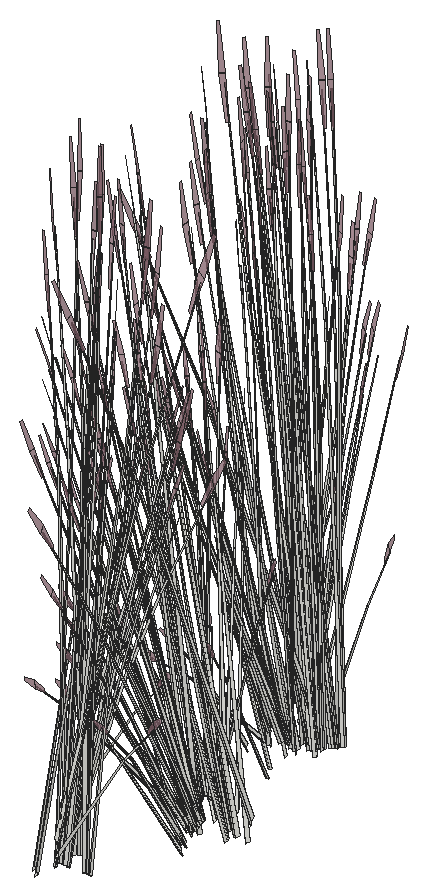
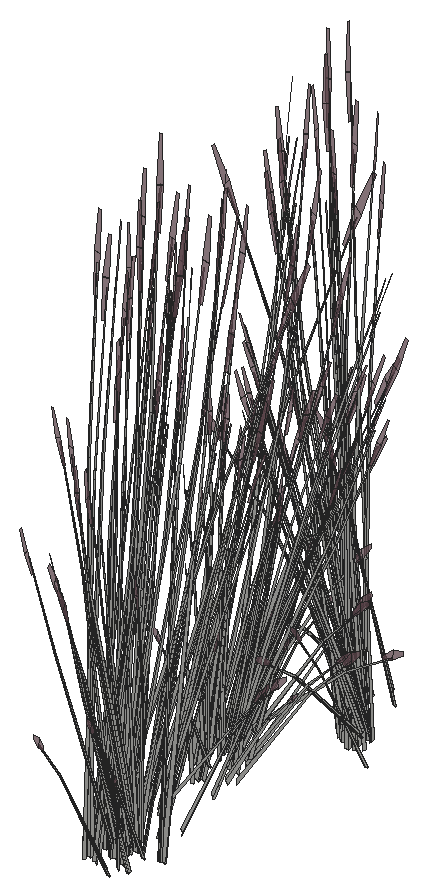
# SketchUp Ruby script. Lengths in inches.
U = 1.inch
M = Sketchup.active_model
def pt(a) = Geom::Point3d.new(a.map { |v| v * U })
def face(e, loops, mat)
  f = e.add_face(loops[0].map { |a| pt(a) })
  loops[1..].each { |l| e.add_face(l.map { |a| pt(a) }).erase! }
  f.material = f.back_material = mat if mat
  f
end
# faces: each face lists its corners as indices into pts; further lists are holes
def faces(e, pts, list, mat = nil) = list.each { |f| face(e, (f[0].is_a?(Array) ? f : [f]).map { |l| l.map { |i| pts[i] } }, mat) }
# xy, xz, yz: faces in a plane at the given z, y or x. An outline is a flat list of corners, or four numbers for a rectangle; further outlines are holes
def ring(l) = l.size == 4 ? [[l[0], l[1]], [l[2], l[1]], [l[2], l[3]], [l[0], l[3]]] : l.each_slice(2).to_a
def flat(e, list, mat, &to3) = list.each { |f| face(e, (f[0].is_a?(Array) ? f : [f]).map { |l| ring(l).map { |u, v| to3.(u, v) } }, mat) }
def xy(e, z, list, mat = nil) = flat(e, list, mat) { |x, y| [x, y, z] }
def xz(e, y, list, mat = nil) = flat(e, list, mat) { |x, z| [x, y, z] }
def yz(e, x, list, mat = nil) = flat(e, list, mat) { |y, z| [x, y, z] }
def lines(e, pts, list) = list.each { |a, b| e.add_line(pt(pts[a]), pt(pts[b])) }
# prism: a flat outline (further loops are holes) pulled along v
def prism(e, loops, v, mat = nil)
  f = face(e, loops, mat); d = Geom::Vector3d.new(v.map { |x| x * U })
  f.pushpull(f.normal.samedirection?(d) ? d.length : -d.length)
end
def box(e, o, s, mat = nil) = prism(e, [[o, [o[0] + s[0], o[1], o[2]], [o[0] + s[0], o[1] + s[1], o[2]], [o[0], o[1] + s[1], o[2]]]], [0, 0, s[2]], mat)
def at(x, y, z, deg = 0) = Geom::Transformation.translation(pt([x, y, z])) * Geom::Transformation.rotation(ORIGIN, Z_AXIS, deg.degrees)
def axes(o, x, y, z) = Geom::Transformation.new([*x, 0, *y, 0, *z, 0, *pt(o).to_a, 1])
def part(name) = M.definitions.add(name)
# library, detail: a bought-in or finely detailed component or shape, given as its bounding box
def library(name, o, s) = part(name).tap { |d| box(d.entities, o, s) }
def detail(e, o, s) = box(e.add_group.entities, o, s)
def put(e, d, t, mat = nil) = e.add_instance(d, t).tap { |i| i.material = mat if mat }
def group(e, t, mat = nil) = e.add_group.tap { |g| g.transformation = t; g.material = mat if mat }.entities
root = M.entities
M.materials.add("LightPink_Translucent").color = [144, 107, 117]
M.materials["LightPink_Translucent"].alpha = 0.75
c1 = part("blade")
p = [[2.15,0.21,22],[0,0.17,0],[0.09,0.45,0],[2.18,0.31,22],[2.29,0.31,22],[0.38,0.45,0],
  [2.48,0.24,33],[2.49,0.24,33],[2.48,0.22,33]]
faces(c1.entities,p,[[0,1,2,3],[4,5,2,3],[6,3,4,7],[8,0,3,6]])
c2 = part("seeds")
p = [[0.3,-0.1,1.38],[-0.01,-0.03,1.59],[-0.01,-0.03,0.03],[0.14,-0.07,-0.07],[0.29,-0.03,3],[0.15,0.01,3.11]]
faces(c2.entities,p,[[0,1,2,3],[1,0,4,5]],"LightPink_Translucent")
c3 = part("blade with seeds")
put(c3.entities,c1,at(0,0,0))
put(c3.entities,c2,axes([2.4,0.25,30.99],[1.5799,-0.05474,1.17369],[-0.12525,1.92788,0.29478],[-0.07173,-0.02425,1.56792]))
put(root,c3,axes([290.45,481.91,3.875],[-0.0219,-0.25042,1.71376],[0.94901,0.16613,0.13857],[-0.0587,0.35688,0.73262]))
put(root,c3,axes([289.3,486.41,2.72],[0.43405,-0.58792,0.44739],[0.90188,0.28295,-0.21531],[0,0.13553,1.43643]))
put(root,c3,axes([289.13,486.75,2.29],[0,0.75458,-0.05637],[-1.11865,0,0],[0,0.02371,1.79368]))
put(root,c3,axes([289.22,486.21,2.21],[0.53742,0.54764,-0.44739],[-0.81403,0.38564,0.21531],[0.17391,0.06776,1.43643]))
put(root,c3,axes([291.58,486.74,2.48],[0,-0.65246,0.49651],[1.00089,0,0],[0,0.1486,1.57504]))
put(root,c3,axes([289.07,487.23,2.72],[0.97146,-0.04028,0.44739],[0.08785,0.66859,-0.21531],[-0.17391,0.06776,1.43643]))
put(root,c3,axes([289.68,486.54,2.62],[0.83351,-0.19028,0.1448],[0.29189,0.54335,-0.41347],[0,0.11958,1.26744]))
put(root,c3,axes([290.67,484.2,4.72],[0.1134,0.10507,1.74944],[0.91515,0.04128,-0.27667],[0.09203,0.23172,0.14031]))
put(root,c3,axes([288.92,488.45,2.2],[0.90188,0.29293,0],[-0.43405,0.60866,0],[0,0,1.74954]))
put(root,c3,axes([289.2,483.19,3.36],[0.01966,-0.33682,1.54345],[0.88405,0.17791,0.21329],[-0.0766,0.35897,0.72882]))
put(root,c3,axes([295.84,495.1,3.875],[0.2045,0.20949,1.71376],[-0.94495,0.17636,0.13857],[-0.21357,-0.32887,0.73262]))
put(root,c3,axes([289.79,488.72,2.48],[0.83726,-0.32623,0.49651],[0.50045,0.58498,0],[-0.19069,0.0743,1.57504]))
put(root,c3,axes([288.6,488.21,2.29],[0.38895,0.74956,-0.06012],[-1.11135,0.26265,0],[0.01358,0.02618,1.72173]))
put(root,c3,axes([295.58,494.55,2.59],[-0.05417,0.21344,1.43002],[-0.79196,0.17867,-0.30754],[-0.18512,-0.27588,0.61141]))
put(root,c3,axes([291.8125,487.22,2.2],[-1.1181,-0.00522,-0.04976],[0,-0.72922,0.49943],[-0.03514,0.166,1.58352]))
put(root,c3,axes([289.39,486.59,2.67],[1.00749,0.31132,-0.29095],[-0.48511,0.65709,-0.50002],[0.03166,0.16133,1.59708]))
put(root,c3,axes([291.58,487.33,2.03],[-0.62448,0.40708,-0.30978],[-0.62448,-0.40708,0.30978],[0,0.13112,1.38974]))
put(root,c3,axes([289.28,487.08,2.21],[-0.43405,0.58792,-0.44739],[-0.90188,-0.28295,0.21531],[0,0.13553,1.43643]))
put(root,c3,axes([289.04,488.96,5.05],[-0.13817,-0.52554,0.35414],[0.78985,-0.13877,-0.4572],[0.21215,0.1506,0.87481]))
put(root,c3,axes([289.31,488.76,2.33],[1.11998,0.21207,0.30756],[-0.2802,0.75803,-0.36492],[-0.18537,0.09487,1.64885]))
put(root,c3,axes([296.46,493.41,4.71],[-0.01669,0.07821,1.77383],[-0.82314,0.28383,-0.16761],[-0.24223,-0.14508,0.31391]))
put(root,c3,axes([292.01,487.34,2.02],[0,0.65246,-0.49651],[-1.00089,0,0],[0,0.1486,1.57504]))
put(root,c3,axes([289.57,485.9375,4.47],[-0.77304,-0.33901,1.38283],[0.81626,-0.52782,0.59665],[0.24941,0.31809,1.33663]))
put(root,c3,axes([295.31,494.2,2.77],[0.46666,0.22709,1.1486],[-0.67962,0.13651,0.84392],[-0.14541,-0.17452,0.25299]))
put(root,c3,axes([296.43,495.41,4.98],[-0.76283,-0.31537,-0.71045],[0.54213,-0.55263,0.08574],[-0.27638,-0.1883,1.00501]))
put(root,c3,axes([296.17,494.99,4.53],[-0.13817,-0.52554,-0.35414],[0.78985,-0.13877,0.4572],[-0.21215,-0.1506,0.87481]))
put(root,c3,axes([289.79,487.25,2.09],[0.32803,0.59738,-0.69212],[-0.94492,0.21515,-0.18165],[0.03626,0.20229,1.52773]))
put(root,c3,axes([294.9375,494.89,1.49],[-0.08666,0.08595,1.76342],[-0.87574,0.18531,-0.26939],[-0.21156,-0.16858,0.30037]))
put(root,c3,axes([287.15,489.04,5.05],[0.2697,-0.50175,0.35414],[0.78684,0.14635,-0.4572],[0.07215,0.20201,0.87481]))
put(root,c3,axes([289.16,489.4375,4.73],[-0.4066,0.41448,0.0643],[-0.57901,-0.24131,0.50621],[0.18719,0.13288,0.77189]))
put(root,c3,axes([296.08,495.42,4.68],[-0.88277,0.1551,-0.51099],[-0.15442,-0.58737,-0.3958],[-0.23711,-0.16832,0.97773]))
put(root,c3,axes([288.21,490.83,5.65],[0.61821,-0.37431,-0.06488],[0.56645,0.40995,-0.29416],[0.03988,0.11616,0.97024]))
put(root,c3,axes([296.7,494.9,5.43],[-0.59706,0.6255,-0.13619],[-0.86465,-0.36036,-0.75594],[-0.30056,-0.17672,1.14864]))
put(root,c3,axes([289.34,489.32,4.73],[-0.88979,0.14973,0.48003],[-0.15442,-0.58737,0.3958],[0.20926,0.17311,0.9933]))
put(root,c3,axes([286.89,489.25,5.03],[0.87543,-0.30377,-0.1216],[0.4302,0.53915,-0.67495],[0.1155,0.2272,1.02557]))
put(root,c3,axes([294.41,494.72,4.72],[-0.19249,-0.00461,1.74944],[-0.61281,0.46055,-0.27667],[-0.32697,-0.0941,0.14031]))
put(root,c3,axes([287.05,489.37,1.49],[0.14478,-0.0355,1.76342],[0.8709,0.19542,-0.26939],[0.02547,0.22025,0.30037]))
put(root,c3,axes([298.26,498.97,3.33],[0.77308,0.2631,1.51261],[-0.75736,0.56681,0.59816],[-0.33924,-0.33594,1.26806]))
put(root,c3,axes([296.64,495.42,5.05],[0.13817,0.52554,0.35414],[-0.78985,0.13877,-0.4572],[-0.21215,-0.1506,0.87481]))
put(root,c3,axes([294.27,495.76,5.09],[0.7388,-0.48151,0.53763],[0.63717,0.51135,0.4433],[-0.34662,-0.08882,1.11249]))
put(root,c3,axes([287.64,489.23,4.68],[0.87941,0.16356,-0.51099],[-0.30143,0.56078,-0.3958],[0.08064,0.22578,0.97773]))
put(root,c3,axes([288.14,488.07,3.875],[-0.2045,-0.20949,1.71376],[0.94495,-0.17636,0.13857],[0.21357,0.32887,0.73262]))
put(root,c3,axes([287.24,489.57,4.53],[-0.2697,0.50175,-0.35414],[-0.78684,-0.14635,0.4572],[0.07215,0.20201,0.87481]))
put(root,c3,axes([294.6,495.76,4.73],[0.04505,-0.49615,0.0643],[0.68022,0.0136,0.50621],[-0.26056,-0.05192,0.77189]))
put(root,c3,axes([294.34,495.91,4.53],[-0.50902,-0.40851,-0.35414],[0.58122,-0.38671,0.4572],[-0.29531,-0.05884,0.87481]))
put(root,c3,axes([294.4,495.22,2.13],[-0.25807,0.53277,-0.03893],[-0.79428,-0.16389,-0.17649],[-0.1206,-0.08714,0.58215]))
put(root,c3,axes([293.97,497.65,2.375],[-1.11865,0,0],[0,-0.72922,-0.51607],[0,-0.16609,1.63711]))
put(root,c3,axes([287.32,489.12,4.98],[0.42698,0.53052,-0.71045],[-0.87893,0.29566,0.08574],[0.09984,0.25633,1.00501]))
put(root,c3,axes([286.68,490.46,4.72],[0.1134,0.10507,1.74944],[0.91515,0.04128,-0.27667],[0.09203,0.23172,0.14031]))
put(root,c3,axes([294.84,497.46,2.33],[-0.83213,0.54855,0.30756],[-0.83263,-0.54278,-0.36492],[-0.02906,-0.15578,1.64885]))
put(root,c3,axes([293.67,495.11,4.71],[0.06632,0.06511,1.77383],[-0.31973,0.58531,-0.16761],[-0.32381,0.00424,0.31391]))
put(root,c3,axes([294.58,496.32,4.68],[-0.6496,0.4322,-0.51099],[-0.5689,-0.45657,-0.3958],[-0.33005,-0.06576,0.97773]))
put(root,c3,axes([295.0625,496.125,5.05],[0.50902,0.40851,0.35414],[-0.58122,0.38671,-0.4572],[-0.29531,-0.05884,0.87481]))
put(root,c3,axes([293.12,496.89,2.77],[0.57115,-0.04669,1.1486],[-0.36229,0.41137,0.84392],[-0.28224,-0.06171,0.25299]))
put(root,c3,axes([294.92,495.87,5.03],[-0.0479,0.66354,-0.1216],[-0.90696,-0.01814,-0.67495],[-0.3493,-0.04609,1.02557]))
put(root,c3,axes([296.53,498.5,2.06],[-0.9306,-0.10697,-0.62353],[0.19638,-0.65984,-0.16365],[-0.27771,-0.07995,1.37633]))
put(root,c3,axes([293.62,497.26,4.73],[0.25275,-0.59491,0.48003],[0.83094,0.20343,0.3958],[-0.32677,0.03575,0.9933]))
put(root,c3,axes([293.55,497.11,4.73],[-0.32857,-0.44488,0.0643],[0.59916,-0.21775,0.50621],[-0.26412,0.04296,0.77189]))
put(root,c3,axes([293.54,497.5625,1.49],[0.02269,0.10283,1.76342],[-0.45738,0.53699,-0.26939],[-0.32488,-0.02707,0.30037]))
put(root,c3,axes([295.54,499.5,2.03],[-0.21015,-0.56852,-0.30978],[0.83462,-0.16144,0.30978],[-0.16826,-0.06556,1.38974]))
put(root,c3,axes([295.31,499.75,2.02],[-0.83726,-0.32623,-0.49651],[0.50045,-0.58498,0],[-0.19069,-0.0743,1.57504]))
put(root,c3,axes([297.58,498.59,2.67],[-0.90324,0.43318,-0.29095],[-0.60064,-0.61207,-0.50002],[-0.22285,-0.06216,1.59708]))
put(root,c3,axes([294.23,497.27,5.05],[0.74348,0.18202,0.35414],[-0.21685,0.53102,-0.4572],[-0.29933,0.04869,0.87481]))
put(root,c3,axes([293.95,497.6,4.68],[-0.24236,0.59349,-0.51099],[-0.83094,-0.20343,-0.3958],[-0.33455,0.05442,0.97773]))
put(root,c3,axes([293.91,497.09,5.03],[0.45012,0.59081,-0.1216],[-0.79888,0.29033,-0.67495],[-0.33665,0.07795,1.02557]))
put(root,c3,axes([295.82,500.14,2.375],[-0.55932,0.6538,0],[-0.93577,-0.36461,-0.51607],[-0.21313,-0.08304,1.63711]))
put(root,c3,axes([293.82,498.75,4.73],[-0.22187,-0.60049,0.48003],[0.87033,-0.10422,0.3958],[-0.25651,0.14123,0.9933]))
put(root,c3,axes([293.64,498.63,4.73],[-0.61415,-0.2744,0.0643],[0.35756,-0.39076,0.50621],[-0.1969,0.12633,0.77189]))
put(root,c3,axes([294.35,498.55,5.05],[0.77872,-0.09325,0.35414],[0.20563,0.53305,-0.4572],[-0.22316,0.14318,0.87481]))
put(root,c3,axes([291.35,498.31,4.71],[0.11417,0.0175,1.77383],[0.35319,0.57649,-0.16761],[-0.23371,0.15131,0.31391]))
put(root,c3,axes([292.31,500.14,2.77],[0.37283,-0.29571,1.1486],[0.14711,0.46813,0.84392],[-0.26943,0.08382,0.25299]))
put(root,c3,axes([293.72,498.86,4.53],[-0.77872,0.09325,-0.35414],[-0.20563,-0.53305,0.4572],[-0.22316,0.14318,0.87481]))
put(root,c3,axes([292.58,500.06,5.65],[0.78943,0.17416,-0.06488],[-0.24284,0.53604,-0.29416],[-0.12912,0.08139,0.97024]))
put(root,c3,axes([298.18,499.07,2.06],[-0.60257,0.49041,-0.62353],[-0.74854,-0.44469,-0.16365],[-0.24146,0.12234,1.37633]))
put(root,c3,axes([293.95,498.5,5.03],[0.82753,0.35977,-0.1216],[-0.47675,0.52101,-0.67495],[-0.2338,0.18111,1.02557]))
put(root,c3,axes([295.06,498.34,3.875],[0.22344,-0.20048,1.71376],[0.56419,0.54113,0.13857],[-0.38697,0.24643,0.73262]))
put(root,c3,axes([294.36,498.92,4.68],[0.22982,0.59576,-0.51099],[-0.87033,0.10422,-0.3958],[-0.24941,0.16002,0.97773]))
put(root,c3,axes([294.85,499.92,4.73],[-0.73517,-0.0304,0.0643],[0.02016,-0.45906,0.50621],[-0.07693,0.17585,0.77189]))
put(root,c3,axes([293.29,500.44,1.49],[0.12,0.06519,1.76342],[0.20347,0.60397,-0.26939],[-0.26596,0.12879,0.30037]))
put(root,c3,axes([295.09,499.96,4.73],[-0.63704,-0.44518,0.48003],[0.67652,-0.38394,0.3958],[-0.11751,0.20886,0.9933]))
put(root,c3,axes([294.89,498.83,3.875],[0.16657,-0.22426,1.71376],[0.69879,0.4641,0.13857],[-0.31524,0.28926,0.73262]))
put(root,c3,axes([292.3,508.18,4.72],[-0.13683,-0.09148,1.74944],[-0.91315,0.058,-0.27667],[-0.14574,-0.2188,0.14031]))
put(root,c3,axes([295.09,500.1,4.53],[-0.60531,0.34352,-0.35414],[-0.573,-0.39225,0.4572],[-0.08718,0.19929,0.87481]))
put(root,c3,axes([293,499.99,4.72],[-0.02224,0.12912,1.74944],[0.63107,0.44917,-0.27667],[-0.16521,0.21241,0.14031]))
put(root,c3,axes([293.26,509.72,4.98],[-0.42698,-0.53052,-0.71045],[0.87893,-0.29566,0.08574],[-0.09984,-0.25633,1.00501]))
put(root,c3,axes([292.52,508.54,1.49],[-0.15005,0.02351,1.76342],[-0.82981,-0.26461,-0.26939],[0.01392,-0.22072,0.30037]))
put(root,c3,axes([293.34,509.27,4.53],[0.2697,-0.50175,-0.35414],[0.78684,0.14635,0.4572],[-0.07215,-0.20201,0.87481]))
put(root,c3,axes([292.9375,509.61,4.68],[-0.87941,-0.16356,-0.51099],[0.30143,-0.56078,-0.3958],[-0.08064,-0.22578,0.97773]))
put(root,c3,axes([292.93,501.32,4.71],[0.10149,-0.03939,1.77383],[0.83886,0.26202,-0.16761],[-0.01971,0.21816,0.31391]))
put(root,c3,axes([291.18,509.26,5.09],[0.99656,-0.1677,0.53763],[0.17295,0.65785,0.4433],[-0.23438,-0.19388,1.11249]))
put(root,c3,axes([293.69,509.59,5.03],[-0.87543,0.30377,-0.1216],[-0.4302,-0.53915,-0.67495],[-0.1155,-0.2272,1.02557]))
put(root,c3,axes([290.21,508.67,2.77],[0.46666,0.22709,1.1486],[-0.67962,0.13651,0.84392],[-0.14541,-0.17452,0.25299]))
put(root,c3,axes([294.8,501.09,2.59],[0.28231,-0.10293,1.43002],[0.69701,0.31035,-0.30754],[-0.20746,0.26854,0.61141]))
put(root,c3,axes([291.41,509.41,4.73],[0.4066,-0.41448,0.0643],[0.57901,0.24131,0.50621],[-0.18719,-0.13288,0.77189]))
put(root,c3,axes([291.28,511.71,2.1],[-0.36739,-0.66907,-0.69835],[1.05831,-0.24096,-0.18329],[-0.04061,-0.22656,1.54149]))
put(root,c3,axes([293.43,509.8,5.05],[-0.2697,0.50175,0.35414],[-0.78684,-0.14635,-0.4572],[-0.07215,-0.20201,0.87481]))
put(root,c3,axes([292.37,509,2.13],[-0.61821,0.37431,-0.03893],[-0.56645,-0.40995,-0.17649],[-0.03988,-0.11616,0.58215]))
put(root,c3,axes([293.16,513.4375,3.33],[0.77308,0.2631,1.51261],[-0.75736,0.56681,0.59816],[-0.33924,-0.33594,1.26806]))
put(root,c3,axes([291.54,509.88,5.05],[0.13817,0.52554,0.35414],[-0.78985,0.13877,-0.4572],[-0.21215,-0.1506,0.87481]))
put(root,c3,axes([289.12,511.62,2.02],[0,-0.65246,-0.49651],[1.00089,0,0],[0,-0.1486,1.57504]))
put(root,c3,axes([291.84,511.89,2.21],[0.43405,-0.58792,-0.44739],[0.90188,0.28295,0.21531],[0,-0.13553,1.43643]))
put(root,c3,axes([289.55,511.63,2.03],[0.62448,-0.40708,-0.30978],[0.62448,0.40708,0.30978],[0,-0.13112,1.38974]))
put(root,c3,axes([291.73,512.375,2.67],[-1.00749,-0.31132,-0.29095],[0.48511,-0.65709,-0.50002],[-0.03166,-0.16133,1.59708]))
put(root,c3,axes([289.74,511.92,2.33],[-0.83213,0.54855,0.30756],[-0.83263,-0.54278,-0.36492],[-0.02906,-0.15578,1.64885]))
put(root,c3,axes([291.99,513.07,2.4375],[0.23711,-0.77313,-0.23429],[1.12425,0.13477,0.51271],[-0.19645,-0.10677,1.5644]))
put(root,c3,axes([289.55,512.23,2.48],[0,0.65246,0.49651],[-1.00089,0,0],[0,-0.1486,1.57504]))
put(root,c3,axes([291.91,512.75,2.21],[-0.53742,-0.54764,-0.44739],[0.81403,-0.38564,0.21531],[-0.17391,-0.06776,1.43643]))
put(root,c3,axes([292.02,511.98,2.36],[0.38895,0.72959,0.45755],[-1.11135,0.2537,0.17955],[0.01358,-0.13406,1.58856]))
put(root,c3,axes([291.83,512.55,2.72],[-0.43405,0.58792,0.44739],[-0.90188,-0.28295,-0.21531],[0,-0.13553,1.43643]))
put(root,c3,axes([293.7,512.625,2.3],[-0.83213,-0.56158,-0.06131],[0.83263,-0.56193,0],[-0.02906,-0.01961,1.75571]))
put(root,c3,axes([292.12,512.69,2.36],[1.13071,0.13747,0.45755],[-0.23011,0.77639,0.17955],[-0.16524,-0.07497,1.58856]))
put(root,c3,axes([291.51,513.93,2.47],[0.96132,-0.17317,0.17642],[0.23737,0.64447,0.35086],[-0.08574,-0.0939,1.60407]))
put(root,c3,axes([292.95,513.78,2.2],[-0.29189,-0.56252,0],[0.83351,-0.19699,0],[0,0,1.54371]))
put(root,c3,axes([292.4,513.25,2.62],[-0.17258,0.58229,0.1448],[-0.84319,-0.10108,-0.41347],[-0.15345,-0.05979,1.26744]))
put(root,c3,axes([294.37,513.97,2.47],[0.25843,-0.64844,0.17642],[0.9457,0.1835,0.35086],[-0.16336,0.00316,1.60407]))
put(root,c3,axes([292.75,514.04,2.2],[-0.90188,-0.29293,0],[0.43405,-0.60866,0],[0,0,1.62707]))
put(root,c3,axes([293.5,513.26,2.46],[-0.87356,-0.52515,-0.25192],[0.73507,-0.5897,0.5513],[-0.23523,0.06143,1.68216]))
put(root,c3,axes([291.2,514.26,2.48],[0.83726,0.32623,0.49651],[-0.50045,0.58498,0],[-0.19069,-0.0743,1.57504]))
put(root,c3,axes([293.92,512.82,2.72],[0.97146,-0.04028,0.44739],[0.08785,0.66859,-0.21531],[-0.17391,0.06776,1.43643]))
put(root,c3,axes([293.06,513.15,2.21],[-0.97146,0.04028,-0.44739],[-0.08785,-0.66859,0.21531],[-0.17391,0.06776,1.43643]))
put(root,c3,axes([294.13,514.7,2.19],[-0.55235,-0.65609,-0.05142],[0.93577,-0.36461,0.51607],[-0.23059,0.06247,1.6363]))
put(root,c3,axes([293.9375,513.11,2.62],[0.66093,0.39201,0.1448],[-0.5513,0.44227,-0.41347],[-0.15345,0.05979,1.26744]))
put(root,c3,axes([294.64,514.32,2.48],[0.83726,-0.32623,0.49651],[0.50045,0.58498,0],[-0.19069,0.0743,1.57504]))
put(root,c3,axes([293.88,514.61,2.03],[-0.83462,-0.16144,-0.30978],[0.21015,-0.56852,0.30978],[-0.16826,0.06556,1.38974]))
put(root,c3,axes([293.74,512.96,2.67],[0.10425,0.7445,-0.29095],[-1.08575,0.04502,-0.50002],[-0.19119,0.09917,1.59708]))
put(root,c3,axes([293.08,513.53,2.06],[-0.60257,0.49041,-0.62353],[-0.74854,-0.44469,-0.16365],[-0.24146,0.12234,1.37633]))
put(root,c3,axes([294.16,514.36,2.33],[1.11998,0.21207,0.30756],[-0.2802,0.75803,-0.36492],[-0.18537,0.09487,1.64885]))
put(root,c3,axes([294.08,514.87,2.02],[-0.83726,0.32623,-0.49651],[-0.50045,-0.58498,0],[-0.19069,0.0743,1.57504]))
put(root,c3,axes([290.3,514.07,5.05],[0.60531,-0.34352,0.35414],[0.573,0.39225,-0.4572],[-0.08718,0.19929,0.87481]))
put(root,c3,axes([294.84,514.77,2.375],[0.55932,0.6538,0],[-0.93577,0.36461,-0.51607],[-0.21313,0.08304,1.63711]))
put(root,c3,axes([294.36,512.18,2.84],[-0.02444,-0.61432,1.41272],[1.10603,0.15924,0.59816],[-0.26159,0.33615,1.3335]))
put(root,c3,axes([289.75,514.39,4.73],[-0.73517,-0.0304,0.0643],[0.02016,-0.45906,0.50621],[-0.07693,0.17585,0.77189]))
put(root,c3,axes([291.76,515.09,4.73],[-0.6592,0.22175,0.0643],[-0.32265,-0.40436,0.50621],[0.06366,0.17825,0.77189]))
put(root,c3,axes([289.99,514.5625,4.53],[-0.60531,0.34352,-0.35414],[-0.573,-0.39225,0.4572],[-0.08718,0.19929,0.87481]))
put(root,c3,axes([289.92,514.17,5.4],[0.98321,0.03233,-0.13498],[-0.02687,0.61208,-0.74919],[-0.0683,0.23574,1.13838]))
put(root,c3,axes([291.99,515.05,5.0625],[-0.88151,-0.17057,0.53283],[0.30143,-0.56078,0.43934],[0.05297,0.22053,1.10256]))
put(root,c3,axes([290.37,515.9,2.77],[-0.02315,-0.38796,1.1486],[0.57853,0.27671,0.84392],[-0.11378,0.18492,0.25299]))
put(root,c3,axes([291.89,514.97,1.49],[0.14478,-0.0355,1.76342],[0.8709,0.19542,-0.26939],[0.02547,0.22025,0.30037]))
put(root,c3,axes([290.59,514.4,5],[0.64041,0.4384,-0.5672],[-0.67652,0.38394,-0.43934],[-0.09744,0.22274,1.08528]))
put(root,c3,axes([289.89,515.06,2.82],[0.8127,-0.11554,0.06507],[0.18684,0.46549,-0.86304],[-0.05152,0.23564,0.7736]))
put(root,c3,axes([292.09,515.17,4.53],[-0.2697,0.50175,-0.35414],[-0.78684,-0.14635,0.4572],[0.07215,0.20201,0.87481]))
put(root,c3,axes([290.39,514.2,5.34],[-0.02328,0.60353,-0.7886],[-0.98022,-0.04053,0.09517],[-0.10344,0.25568,1.11556]))
put(root,c3,axes([287.83,515.78,4.71],[0.10149,-0.03939,1.77383],[0.83886,0.26202,-0.16761],[-0.01971,0.21816,0.31391]))
put(root,c3,axes([291.32,513.77,3.875],[-0.0219,-0.25042,1.71376],[0.94901,0.16613,0.13857],[-0.0587,0.35688,0.73262]))
put(root,c3,axes([290.0625,515.05,3.36],[0.01966,-0.33682,1.54345],[0.88405,0.17791,0.21329],[-0.0766,0.35897,0.72882]))
